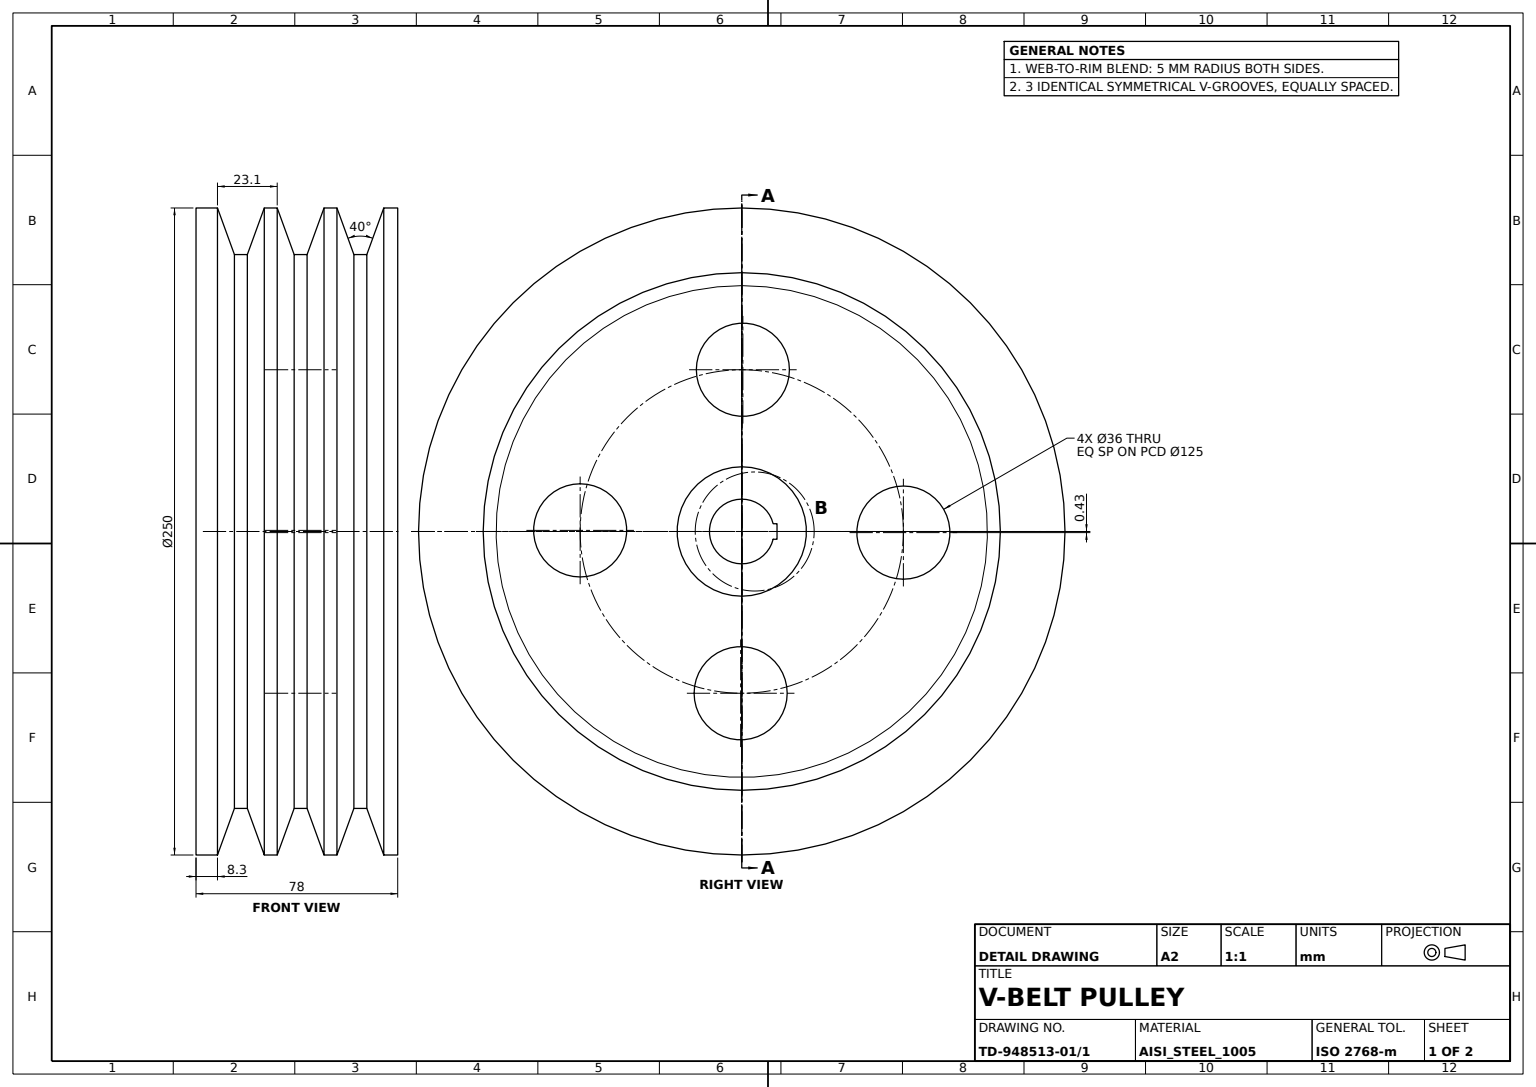
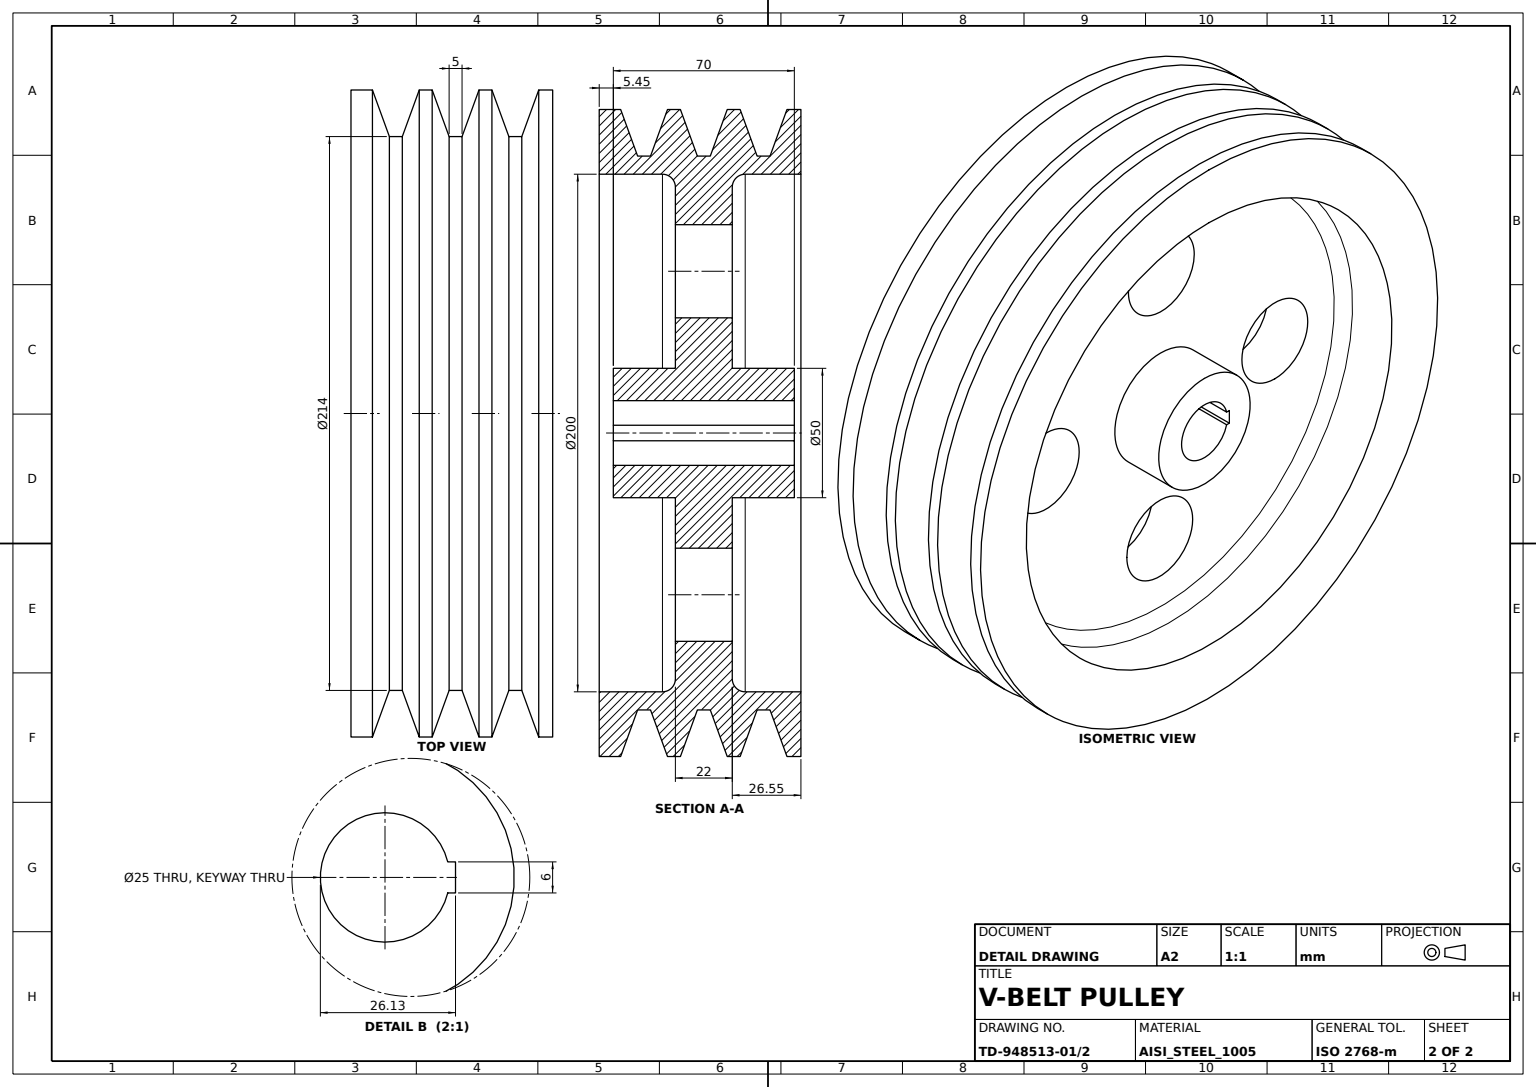
ISO-10303-21;
HEADER;
FILE_DESCRIPTION((''),'2;1');
FILE_NAME('','',(''),(''),'','','');
FILE_SCHEMA(('AUTOMOTIVE_DESIGN'));
ENDSEC;
DATA;
#1=APPLICATION_CONTEXT('');
#2=PRODUCT_CONTEXT('',#1,'mechanical');
#3=PRODUCT('','','',(#2));
#4=PRODUCT_DEFINITION_FORMATION('','',#3);
#5=PRODUCT_DEFINITION_CONTEXT('',#1,'design');
#6=PRODUCT_DEFINITION('','',#4,#5);
#7=PRODUCT_DEFINITION_SHAPE('','',#6);
#8=(LENGTH_UNIT()NAMED_UNIT(*)SI_UNIT(.MILLI.,.METRE.));
#9=(NAMED_UNIT(*)PLANE_ANGLE_UNIT()SI_UNIT($,.RADIAN.));
#10=(NAMED_UNIT(*)SI_UNIT($,.STERADIAN.)SOLID_ANGLE_UNIT());
#11=UNCERTAINTY_MEASURE_WITH_UNIT(LENGTH_MEASURE(0.005),#8,'distance_accuracy_value','');
#12=(GEOMETRIC_REPRESENTATION_CONTEXT(3)GLOBAL_UNCERTAINTY_ASSIGNED_CONTEXT((#11))GLOBAL_UNIT_ASSIGNED_CONTEXT((#8,#9,#10))REPRESENTATION_CONTEXT('',''));
#13=CARTESIAN_POINT('',(35.,12.134661,-3.));
#14=VERTEX_POINT('',#13);
#15=CARTESIAN_POINT('',(35.,13.634661,-3.));
#16=VERTEX_POINT('',#15);
#17=DIRECTION('',(0.,1.,0.));
#18=VECTOR('',#17,1000.);
#19=LINE('',#13,#18);
#20=EDGE_CURVE('',#14,#16,#19,.T.);
#21=ORIENTED_EDGE('',*,*,#20,.F.);
#22=CARTESIAN_POINT('',(35.,12.134661,3.));
#23=VERTEX_POINT('',#22);
#24=CARTESIAN_POINT('',(35.,0.,0.));
#25=DIRECTION('',(-1.,0.,0.));
#26=DIRECTION('',(0.,0.,1.));
#27=AXIS2_PLACEMENT_3D('',#24,#25,#26);
#28=CIRCLE('',#27,12.5);
#29=EDGE_CURVE('',#14,#23,#28,.T.);
#30=ORIENTED_EDGE('',*,*,#29,.T.);
#31=CARTESIAN_POINT('',(35.,13.634661,3.));
#32=VERTEX_POINT('',#31);
#33=DIRECTION('',(0.,-1.,0.));
#34=VECTOR('',#33,1000.);
#35=LINE('',#31,#34);
#36=EDGE_CURVE('',#32,#23,#35,.T.);
#37=ORIENTED_EDGE('',*,*,#36,.F.);
#38=VECTOR('',#26,1000.);
#39=LINE('',#15,#38);
#40=EDGE_CURVE('',#16,#32,#39,.T.);
#41=ORIENTED_EDGE('',*,*,#40,.F.);
#42=EDGE_LOOP('',(#21,#30,#37,#41));
#43=FACE_BOUND('',#42,.T.);
#44=CARTESIAN_POINT('',(35.,0.,25.));
#45=VERTEX_POINT('',#44);
#46=CIRCLE('',#27,25.);
#47=EDGE_CURVE('',#45,#45,#46,.T.);
#48=ORIENTED_EDGE('',*,*,#47,.F.);
#49=EDGE_LOOP('',(#48));
#50=FACE_BOUND('',#49,.T.);
#51=CARTESIAN_POINT('',(35.,12.5,0.));
#52=AXIS2_PLACEMENT_3D('',#51,#25,#26);
#53=PLANE('',#52);
#54=ADVANCED_FACE('',(#43,#50),#53,.F.);
#55=CARTESIAN_POINT('',(11.,0.,25.));
#56=VERTEX_POINT('',#55);
#57=CARTESIAN_POINT('',(11.,0.,0.));
#58=AXIS2_PLACEMENT_3D('',#57,#25,#26);
#59=CIRCLE('',#58,25.);
#60=EDGE_CURVE('',#56,#56,#59,.T.);
#61=ORIENTED_EDGE('',*,*,#60,.F.);
#62=EDGE_LOOP('',(#61));
#63=FACE_BOUND('',#62,.T.);
#64=ORIENTED_EDGE('',*,*,#47,.T.);
#65=EDGE_LOOP('',(#64));
#66=FACE_BOUND('',#65,.T.);
#67=CARTESIAN_POINT('',(0.,0.,0.));
#68=AXIS2_PLACEMENT_3D('',#67,#25,#26);
#69=CYLINDRICAL_SURFACE('',#68,25.);
#70=ADVANCED_FACE('',(#63,#66),#69,.T.);
#71=CARTESIAN_POINT('',(-35.,12.134661,-3.));
#72=VERTEX_POINT('',#71);
#73=VECTOR('',#25,1000.);
#74=LINE('',#13,#73);
#75=EDGE_CURVE('',#14,#72,#74,.T.);
#76=ORIENTED_EDGE('',*,*,#75,.F.);
#77=ORIENTED_EDGE('',*,*,#20,.T.);
#78=CARTESIAN_POINT('',(-35.,13.634661,-3.));
#79=VERTEX_POINT('',#78);
#80=LINE('',#15,#73);
#81=EDGE_CURVE('',#79,#16,#80,.F.);
#82=ORIENTED_EDGE('',*,*,#81,.F.);
#83=LINE('',#71,#18);
#84=EDGE_CURVE('',#72,#79,#83,.T.);
#85=ORIENTED_EDGE('',*,*,#84,.F.);
#86=EDGE_LOOP('',(#76,#77,#82,#85));
#87=FACE_BOUND('',#86,.T.);
#88=AXIS2_PLACEMENT_3D('',#13,#26,#33);
#89=PLANE('',#88);
#90=ADVANCED_FACE('',(#87),#89,.T.);
#91=CARTESIAN_POINT('',(-40.451548,0.,125.));
#92=VERTEX_POINT('',#91);
#93=CARTESIAN_POINT('',(-40.451548,0.,0.));
#94=AXIS2_PLACEMENT_3D('',#93,#25,#26);
#95=CIRCLE('',#94,125.);
#96=EDGE_CURVE('',#92,#92,#95,.T.);
#97=ORIENTED_EDGE('',*,*,#96,.T.);
#98=EDGE_LOOP('',(#97));
#99=FACE_BOUND('',#98,.T.);
#100=CARTESIAN_POINT('',(-40.451548,0.,100.));
#101=VERTEX_POINT('',#100);
#102=CIRCLE('',#94,100.);
#103=EDGE_CURVE('',#101,#101,#102,.T.);
#104=ORIENTED_EDGE('',*,*,#103,.F.);
#105=EDGE_LOOP('',(#104));
#106=FACE_BOUND('',#105,.T.);
#107=CARTESIAN_POINT('',(-40.451548,125.,0.));
#108=DIRECTION('',(1.,0.,0.));
#109=DIRECTION('',(0.,0.,-1.));
#110=AXIS2_PLACEMENT_3D('',#107,#108,#109);
#111=PLANE('',#110);
#112=ADVANCED_FACE('',(#99,#106),#111,.F.);
#113=CARTESIAN_POINT('',(16.,0.,100.));
#114=VERTEX_POINT('',#113);
#115=CARTESIAN_POINT('',(16.,0.,0.));
#116=AXIS2_PLACEMENT_3D('',#115,#25,#26);
#117=CIRCLE('',#116,100.);
#118=EDGE_CURVE('',#114,#114,#117,.T.);
#119=ORIENTED_EDGE('',*,*,#118,.T.);
#120=EDGE_LOOP('',(#119));
#121=FACE_BOUND('',#120,.T.);
#122=CARTESIAN_POINT('',(37.548452,0.,100.));
#123=VERTEX_POINT('',#122);
#124=CARTESIAN_POINT('',(37.548452,0.,0.));
#125=AXIS2_PLACEMENT_3D('',#124,#25,#26);
#126=CIRCLE('',#125,100.);
#127=EDGE_CURVE('',#123,#123,#126,.T.);
#128=ORIENTED_EDGE('',*,*,#127,.F.);
#129=EDGE_LOOP('',(#128));
#130=FACE_BOUND('',#129,.T.);
#131=CYLINDRICAL_SURFACE('',#68,100.);
#132=ADVANCED_FACE('',(#121,#130),#131,.F.);
#133=ORIENTED_EDGE('',*,*,#40,.T.);
#134=CARTESIAN_POINT('',(-35.,13.634661,3.));
#135=VERTEX_POINT('',#134);
#136=LINE('',#31,#73);
#137=EDGE_CURVE('',#135,#32,#136,.F.);
#138=ORIENTED_EDGE('',*,*,#137,.F.);
#139=LINE('',#78,#38);
#140=EDGE_CURVE('',#79,#135,#139,.T.);
#141=ORIENTED_EDGE('',*,*,#140,.F.);
#142=ORIENTED_EDGE('',*,*,#81,.T.);
#143=EDGE_LOOP('',(#133,#138,#141,#142));
#144=FACE_BOUND('',#143,.T.);
#145=AXIS2_PLACEMENT_3D('',#15,#33,#109);
#146=PLANE('',#145);
#147=ADVANCED_FACE('',(#144),#146,.T.);
#148=ORIENTED_EDGE('',*,*,#118,.F.);
#149=EDGE_LOOP('',(#148));
#150=FACE_BOUND('',#149,.T.);
#151=CARTESIAN_POINT('',(11.,0.,95.));
#152=VERTEX_POINT('',#151);
#153=CIRCLE('',#58,95.);
#154=EDGE_CURVE('',#152,#152,#153,.F.);
#155=ORIENTED_EDGE('',*,*,#154,.F.);
#156=EDGE_LOOP('',(#155));
#157=FACE_BOUND('',#156,.T.);
#158=TOROIDAL_SURFACE('',#116,95.,5.);
#159=ADVANCED_FACE('',(#150,#157),#158,.F.);
#160=CARTESIAN_POINT('',(-11.,-62.498511,-17.568647));
#161=VERTEX_POINT('',#160);
#162=CARTESIAN_POINT('',(-11.,-62.498511,0.431353));
#163=AXIS2_PLACEMENT_3D('',#162,#108,#109);
#164=CIRCLE('',#163,18.);
#165=EDGE_CURVE('',#161,#161,#164,.F.);
#166=ORIENTED_EDGE('',*,*,#165,.T.);
#167=EDGE_LOOP('',(#166));
#168=FACE_BOUND('',#167,.T.);
#169=CARTESIAN_POINT('',(11.,-62.498511,18.431353));
#170=VERTEX_POINT('',#169);
#171=CARTESIAN_POINT('',(11.,-62.498511,0.431353));
#172=AXIS2_PLACEMENT_3D('',#171,#25,#26);
#173=CIRCLE('',#172,18.);
#174=EDGE_CURVE('',#170,#170,#173,.T.);
#175=ORIENTED_EDGE('',*,*,#174,.F.);
#176=EDGE_LOOP('',(#175));
#177=FACE_BOUND('',#176,.T.);
#178=CARTESIAN_POINT('',(-9.,-62.498511,0.431353));
#179=AXIS2_PLACEMENT_3D('',#178,#25,#26);
#180=CYLINDRICAL_SURFACE('',#179,18.);
#181=ADVANCED_FACE('',(#168,#177),#180,.F.);
#182=CARTESIAN_POINT('',(25.602928,0.,107.));
#183=VERTEX_POINT('',#182);
#184=CARTESIAN_POINT('',(25.602928,0.,0.));
#185=AXIS2_PLACEMENT_3D('',#184,#25,#26);
#186=CIRCLE('',#185,107.);
#187=EDGE_CURVE('',#183,#183,#186,.T.);
#188=ORIENTED_EDGE('',*,*,#187,.T.);
#189=EDGE_LOOP('',(#188));
#190=FACE_BOUND('',#189,.T.);
#191=CARTESIAN_POINT('',(20.602928,0.,107.));
#192=VERTEX_POINT('',#191);
#193=CARTESIAN_POINT('',(20.602928,0.,0.));
#194=AXIS2_PLACEMENT_3D('',#193,#25,#26);
#195=CIRCLE('',#194,107.);
#196=EDGE_CURVE('',#192,#192,#195,.T.);
#197=ORIENTED_EDGE('',*,*,#196,.F.);
#198=EDGE_LOOP('',(#197));
#199=FACE_BOUND('',#198,.T.);
#200=CYLINDRICAL_SURFACE('',#68,107.);
#201=ADVANCED_FACE('',(#190,#199),#200,.T.);
#202=ORIENTED_EDGE('',*,*,#96,.F.);
#203=EDGE_LOOP('',(#202));
#204=FACE_BOUND('',#203,.T.);
#205=CARTESIAN_POINT('',(-32.154393,0.,125.));
#206=VERTEX_POINT('',#205);
#207=CARTESIAN_POINT('',(-32.154393,0.,0.));
#208=AXIS2_PLACEMENT_3D('',#207,#25,#26);
#209=CIRCLE('',#208,125.);
#210=EDGE_CURVE('',#206,#206,#209,.T.);
#211=ORIENTED_EDGE('',*,*,#210,.T.);
#212=EDGE_LOOP('',(#211));
#213=FACE_BOUND('',#212,.T.);
#214=CYLINDRICAL_SURFACE('',#68,125.);
#215=ADVANCED_FACE('',(#204,#213),#214,.T.);
#216=CARTESIAN_POINT('',(-16.,0.,-100.));
#217=VERTEX_POINT('',#216);
#218=CARTESIAN_POINT('',(-16.,0.,0.));
#219=AXIS2_PLACEMENT_3D('',#218,#108,#109);
#220=CIRCLE('',#219,100.);
#221=EDGE_CURVE('',#217,#217,#220,.T.);
#222=ORIENTED_EDGE('',*,*,#221,.F.);
#223=EDGE_LOOP('',(#222));
#224=FACE_BOUND('',#223,.T.);
#225=CARTESIAN_POINT('',(-11.,0.,-95.));
#226=VERTEX_POINT('',#225);
#227=CARTESIAN_POINT('',(-11.,0.,0.));
#228=AXIS2_PLACEMENT_3D('',#227,#108,#109);
#229=CIRCLE('',#228,95.);
#230=EDGE_CURVE('',#226,#226,#229,.F.);
#231=ORIENTED_EDGE('',*,*,#230,.F.);
#232=EDGE_LOOP('',(#231));
#233=FACE_BOUND('',#232,.T.);
#234=TOROIDAL_SURFACE('',#219,95.,5.);
#235=ADVANCED_FACE('',(#224,#233),#234,.F.);
#236=CARTESIAN_POINT('',(-9.051464,0.,125.));
#237=VERTEX_POINT('',#236);
#238=CARTESIAN_POINT('',(-9.051464,0.,0.));
#239=AXIS2_PLACEMENT_3D('',#238,#25,#26);
#240=CIRCLE('',#239,125.);
#241=EDGE_CURVE('',#237,#237,#240,.T.);
#242=ORIENTED_EDGE('',*,*,#241,.F.);
#243=EDGE_LOOP('',(#242));
#244=FACE_BOUND('',#243,.T.);
#245=CARTESIAN_POINT('',(-2.5,0.,107.));
#246=VERTEX_POINT('',#245);
#247=CARTESIAN_POINT('',(-2.5,0.,0.));
#248=AXIS2_PLACEMENT_3D('',#247,#25,#26);
#249=CIRCLE('',#248,107.);
#250=EDGE_CURVE('',#246,#246,#249,.T.);
#251=ORIENTED_EDGE('',*,*,#250,.T.);
#252=EDGE_LOOP('',(#251));
#253=FACE_BOUND('',#252,.T.);
#254=CONICAL_SURFACE('',#248,107.,1.221730476);
#255=ADVANCED_FACE('',(#244,#253),#254,.T.);
#256=CARTESIAN_POINT('',(37.548452,0.,125.));
#257=VERTEX_POINT('',#256);
#258=CIRCLE('',#125,125.);
#259=EDGE_CURVE('',#257,#257,#258,.T.);
#260=ORIENTED_EDGE('',*,*,#259,.T.);
#261=EDGE_LOOP('',(#260));
#262=FACE_BOUND('',#261,.T.);
#263=CARTESIAN_POINT('',(32.154393,0.,125.));
#264=VERTEX_POINT('',#263);
#265=CARTESIAN_POINT('',(32.154393,0.,0.));
#266=AXIS2_PLACEMENT_3D('',#265,#25,#26);
#267=CIRCLE('',#266,125.);
#268=EDGE_CURVE('',#264,#264,#267,.T.);
#269=ORIENTED_EDGE('',*,*,#268,.F.);
#270=EDGE_LOOP('',(#269));
#271=FACE_BOUND('',#270,.T.);
#272=ADVANCED_FACE('',(#262,#271),#214,.T.);
#273=ORIENTED_EDGE('',*,*,#29,.F.);
#274=ORIENTED_EDGE('',*,*,#75,.T.);
#275=CARTESIAN_POINT('',(-35.,12.134661,3.));
#276=VERTEX_POINT('',#275);
#277=CARTESIAN_POINT('',(-35.,0.,0.));
#278=AXIS2_PLACEMENT_3D('',#277,#25,#26);
#279=CIRCLE('',#278,12.5);
#280=EDGE_CURVE('',#72,#276,#279,.T.);
#281=ORIENTED_EDGE('',*,*,#280,.T.);
#282=LINE('',#22,#73);
#283=EDGE_CURVE('',#23,#276,#282,.T.);
#284=ORIENTED_EDGE('',*,*,#283,.F.);
#285=EDGE_LOOP('',(#273,#274,#281,#284));
#286=FACE_BOUND('',#285,.T.);
#287=CYLINDRICAL_SURFACE('',#68,12.5);
#288=ADVANCED_FACE('',(#286),#287,.F.);
#289=CARTESIAN_POINT('',(14.051464,0.,125.));
#290=VERTEX_POINT('',#289);
#291=CARTESIAN_POINT('',(14.051464,0.,0.));
#292=AXIS2_PLACEMENT_3D('',#291,#25,#26);
#293=CIRCLE('',#292,125.);
#294=EDGE_CURVE('',#290,#290,#293,.T.);
#295=ORIENTED_EDGE('',*,*,#294,.F.);
#296=EDGE_LOOP('',(#295));
#297=FACE_BOUND('',#296,.T.);
#298=ORIENTED_EDGE('',*,*,#196,.T.);
#299=EDGE_LOOP('',(#298));
#300=FACE_BOUND('',#299,.T.);
#301=CONICAL_SURFACE('',#194,107.,1.221730476);
#302=ADVANCED_FACE('',(#297,#300),#301,.T.);
#303=CARTESIAN_POINT('',(9.051464,0.,125.));
#304=VERTEX_POINT('',#303);
#305=CARTESIAN_POINT('',(9.051464,0.,0.));
#306=AXIS2_PLACEMENT_3D('',#305,#25,#26);
#307=CIRCLE('',#306,125.);
#308=EDGE_CURVE('',#304,#304,#307,.T.);
#309=ORIENTED_EDGE('',*,*,#308,.F.);
#310=EDGE_LOOP('',(#309));
#311=FACE_BOUND('',#310,.T.);
#312=ORIENTED_EDGE('',*,*,#294,.T.);
#313=EDGE_LOOP('',(#312));
#314=FACE_BOUND('',#313,.T.);
#315=ADVANCED_FACE('',(#311,#314),#214,.T.);
#316=ORIENTED_EDGE('',*,*,#127,.T.);
#317=EDGE_LOOP('',(#316));
#318=FACE_BOUND('',#317,.T.);
#319=ORIENTED_EDGE('',*,*,#259,.F.);
#320=EDGE_LOOP('',(#319));
#321=FACE_BOUND('',#320,.T.);
#322=CARTESIAN_POINT('',(37.548452,100.,0.));
#323=AXIS2_PLACEMENT_3D('',#322,#25,#26);
#324=PLANE('',#323);
#325=ADVANCED_FACE('',(#318,#321),#324,.F.);
#326=ORIENTED_EDGE('',*,*,#241,.T.);
#327=EDGE_LOOP('',(#326));
#328=FACE_BOUND('',#327,.T.);
#329=CARTESIAN_POINT('',(-14.051464,0.,125.));
#330=VERTEX_POINT('',#329);
#331=CARTESIAN_POINT('',(-14.051464,0.,0.));
#332=AXIS2_PLACEMENT_3D('',#331,#25,#26);
#333=CIRCLE('',#332,125.);
#334=EDGE_CURVE('',#330,#330,#333,.T.);
#335=ORIENTED_EDGE('',*,*,#334,.F.);
#336=EDGE_LOOP('',(#335));
#337=FACE_BOUND('',#336,.T.);
#338=ADVANCED_FACE('',(#328,#337),#214,.T.);
#339=CARTESIAN_POINT('',(11.,-18.431353,-62.498511));
#340=VERTEX_POINT('',#339);
#341=CARTESIAN_POINT('',(11.,-0.431353,-62.498511));
#342=AXIS2_PLACEMENT_3D('',#341,#25,#33);
#343=CIRCLE('',#342,18.);
#344=EDGE_CURVE('',#340,#340,#343,.T.);
#345=ORIENTED_EDGE('',*,*,#344,.F.);
#346=EDGE_LOOP('',(#345));
#347=FACE_BOUND('',#346,.T.);
#348=CARTESIAN_POINT('',(-11.,-0.431353,-80.498511));
#349=VERTEX_POINT('',#348);
#350=CARTESIAN_POINT('',(-11.,-0.431353,-62.498511));
#351=AXIS2_PLACEMENT_3D('',#350,#108,#109);
#352=CIRCLE('',#351,18.);
#353=EDGE_CURVE('',#349,#349,#352,.F.);
#354=ORIENTED_EDGE('',*,*,#353,.T.);
#355=EDGE_LOOP('',(#354));
#356=FACE_BOUND('',#355,.T.);
#357=CARTESIAN_POINT('',(-9.,-0.431353,-62.498511));
#358=AXIS2_PLACEMENT_3D('',#357,#25,#26);
#359=CYLINDRICAL_SURFACE('',#358,18.);
#360=ADVANCED_FACE('',(#347,#356),#359,.F.);
#361=CARTESIAN_POINT('',(-11.,0.431353,44.498511));
#362=VERTEX_POINT('',#361);
#363=CARTESIAN_POINT('',(-11.,0.431353,62.498511));
#364=AXIS2_PLACEMENT_3D('',#363,#108,#109);
#365=CIRCLE('',#364,18.);
#366=EDGE_CURVE('',#362,#362,#365,.F.);
#367=ORIENTED_EDGE('',*,*,#366,.F.);
#368=EDGE_LOOP('',(#367));
#369=FACE_BOUND('',#368,.T.);
#370=ORIENTED_EDGE('',*,*,#165,.F.);
#371=EDGE_LOOP('',(#370));
#372=FACE_BOUND('',#371,.T.);
#373=ORIENTED_EDGE('',*,*,#353,.F.);
#374=EDGE_LOOP('',(#373));
#375=FACE_BOUND('',#374,.T.);
#376=CARTESIAN_POINT('',(-11.,62.498511,-18.431353));
#377=VERTEX_POINT('',#376);
#378=CARTESIAN_POINT('',(-11.,62.498511,-0.431353));
#379=AXIS2_PLACEMENT_3D('',#378,#108,#109);
#380=CIRCLE('',#379,18.);
#381=EDGE_CURVE('',#377,#377,#380,.F.);
#382=ORIENTED_EDGE('',*,*,#381,.F.);
#383=EDGE_LOOP('',(#382));
#384=FACE_BOUND('',#383,.T.);
#385=ORIENTED_EDGE('',*,*,#230,.T.);
#386=EDGE_LOOP('',(#385));
#387=FACE_BOUND('',#386,.T.);
#388=CARTESIAN_POINT('',(-11.,0.,25.));
#389=VERTEX_POINT('',#388);
#390=AXIS2_PLACEMENT_3D('',#227,#25,#26);
#391=CIRCLE('',#390,25.);
#392=EDGE_CURVE('',#389,#389,#391,.T.);
#393=ORIENTED_EDGE('',*,*,#392,.F.);
#394=EDGE_LOOP('',(#393));
#395=FACE_BOUND('',#394,.T.);
#396=CARTESIAN_POINT('',(-11.,100.,0.));
#397=AXIS2_PLACEMENT_3D('',#396,#108,#109);
#398=PLANE('',#397);
#399=ADVANCED_FACE('',(#369,#372,#375,#384,#387,#395),#398,.F.);
#400=ORIENTED_EDGE('',*,*,#308,.T.);
#401=EDGE_LOOP('',(#400));
#402=FACE_BOUND('',#401,.T.);
#403=CARTESIAN_POINT('',(2.5,0.,107.));
#404=VERTEX_POINT('',#403);
#405=CARTESIAN_POINT('',(2.5,0.,0.));
#406=AXIS2_PLACEMENT_3D('',#405,#25,#26);
#407=CIRCLE('',#406,107.);
#408=EDGE_CURVE('',#404,#404,#407,.T.);
#409=ORIENTED_EDGE('',*,*,#408,.F.);
#410=EDGE_LOOP('',(#409));
#411=FACE_BOUND('',#410,.T.);
#412=AXIS2_PLACEMENT_3D('',#305,#108,#109);
#413=CONICAL_SURFACE('',#412,125.,1.221730476);
#414=ADVANCED_FACE('',(#402,#411),#413,.T.);
#415=CARTESIAN_POINT('',(-25.602928,0.,107.));
#416=VERTEX_POINT('',#415);
#417=CARTESIAN_POINT('',(-25.602928,0.,0.));
#418=AXIS2_PLACEMENT_3D('',#417,#25,#26);
#419=CIRCLE('',#418,107.);
#420=EDGE_CURVE('',#416,#416,#419,.T.);
#421=ORIENTED_EDGE('',*,*,#420,.T.);
#422=EDGE_LOOP('',(#421));
#423=FACE_BOUND('',#422,.T.);
#424=ORIENTED_EDGE('',*,*,#210,.F.);
#425=EDGE_LOOP('',(#424));
#426=FACE_BOUND('',#425,.T.);
#427=CONICAL_SURFACE('',#418,107.,1.221730476);
#428=ADVANCED_FACE('',(#423,#426),#427,.T.);
#429=ORIENTED_EDGE('',*,*,#103,.T.);
#430=EDGE_LOOP('',(#429));
#431=FACE_BOUND('',#430,.T.);
#432=ORIENTED_EDGE('',*,*,#221,.T.);
#433=EDGE_LOOP('',(#432));
#434=FACE_BOUND('',#433,.T.);
#435=ADVANCED_FACE('',(#431,#434),#131,.F.);
#436=ORIENTED_EDGE('',*,*,#366,.T.);
#437=EDGE_LOOP('',(#436));
#438=FACE_BOUND('',#437,.T.);
#439=CARTESIAN_POINT('',(11.,18.431353,62.498511));
#440=VERTEX_POINT('',#439);
#441=CARTESIAN_POINT('',(11.,0.431353,62.498511));
#442=AXIS2_PLACEMENT_3D('',#441,#25,#17);
#443=CIRCLE('',#442,18.);
#444=EDGE_CURVE('',#440,#440,#443,.T.);
#445=ORIENTED_EDGE('',*,*,#444,.F.);
#446=EDGE_LOOP('',(#445));
#447=FACE_BOUND('',#446,.T.);
#448=CARTESIAN_POINT('',(-9.,0.431353,62.498511));
#449=AXIS2_PLACEMENT_3D('',#448,#25,#26);
#450=CYLINDRICAL_SURFACE('',#449,18.);
#451=ADVANCED_FACE('',(#438,#447),#450,.F.);
#452=CARTESIAN_POINT('',(-20.602928,0.,107.));
#453=VERTEX_POINT('',#452);
#454=CARTESIAN_POINT('',(-20.602928,0.,0.));
#455=AXIS2_PLACEMENT_3D('',#454,#25,#26);
#456=CIRCLE('',#455,107.);
#457=EDGE_CURVE('',#453,#453,#456,.T.);
#458=ORIENTED_EDGE('',*,*,#457,.F.);
#459=EDGE_LOOP('',(#458));
#460=FACE_BOUND('',#459,.T.);
#461=ORIENTED_EDGE('',*,*,#334,.T.);
#462=EDGE_LOOP('',(#461));
#463=FACE_BOUND('',#462,.T.);
#464=AXIS2_PLACEMENT_3D('',#331,#108,#109);
#465=CONICAL_SURFACE('',#464,125.,1.221730476);
#466=ADVANCED_FACE('',(#460,#463),#465,.T.);
#467=ORIENTED_EDGE('',*,*,#174,.T.);
#468=EDGE_LOOP('',(#467));
#469=FACE_BOUND('',#468,.T.);
#470=ORIENTED_EDGE('',*,*,#60,.T.);
#471=EDGE_LOOP('',(#470));
#472=FACE_BOUND('',#471,.T.);
#473=ORIENTED_EDGE('',*,*,#344,.T.);
#474=EDGE_LOOP('',(#473));
#475=FACE_BOUND('',#474,.T.);
#476=ORIENTED_EDGE('',*,*,#444,.T.);
#477=EDGE_LOOP('',(#476));
#478=FACE_BOUND('',#477,.T.);
#479=ORIENTED_EDGE('',*,*,#154,.T.);
#480=EDGE_LOOP('',(#479));
#481=FACE_BOUND('',#480,.T.);
#482=CARTESIAN_POINT('',(11.,62.498511,-18.431353));
#483=VERTEX_POINT('',#482);
#484=CARTESIAN_POINT('',(11.,62.498511,-0.431353));
#485=AXIS2_PLACEMENT_3D('',#484,#25,#109);
#486=CIRCLE('',#485,18.);
#487=EDGE_CURVE('',#483,#483,#486,.T.);
#488=ORIENTED_EDGE('',*,*,#487,.T.);
#489=EDGE_LOOP('',(#488));
#490=FACE_BOUND('',#489,.T.);
#491=CARTESIAN_POINT('',(11.,25.,0.));
#492=AXIS2_PLACEMENT_3D('',#491,#25,#26);
#493=PLANE('',#492);
#494=ADVANCED_FACE('',(#469,#472,#475,#478,#481,#490),#493,.F.);
#495=CARTESIAN_POINT('',(-35.,0.,25.));
#496=VERTEX_POINT('',#495);
#497=CIRCLE('',#278,25.);
#498=EDGE_CURVE('',#496,#496,#497,.T.);
#499=ORIENTED_EDGE('',*,*,#498,.T.);
#500=EDGE_LOOP('',(#499));
#501=FACE_BOUND('',#500,.T.);
#502=ORIENTED_EDGE('',*,*,#140,.T.);
#503=LINE('',#134,#34);
#504=EDGE_CURVE('',#135,#276,#503,.T.);
#505=ORIENTED_EDGE('',*,*,#504,.T.);
#506=ORIENTED_EDGE('',*,*,#280,.F.);
#507=ORIENTED_EDGE('',*,*,#84,.T.);
#508=EDGE_LOOP('',(#502,#505,#506,#507));
#509=FACE_BOUND('',#508,.T.);
#510=CARTESIAN_POINT('',(-35.,25.,0.));
#511=AXIS2_PLACEMENT_3D('',#510,#108,#109);
#512=PLANE('',#511);
#513=ADVANCED_FACE('',(#501,#509),#512,.F.);
#514=ORIENTED_EDGE('',*,*,#408,.T.);
#515=EDGE_LOOP('',(#514));
#516=FACE_BOUND('',#515,.T.);
#517=ORIENTED_EDGE('',*,*,#250,.F.);
#518=EDGE_LOOP('',(#517));
#519=FACE_BOUND('',#518,.T.);
#520=ADVANCED_FACE('',(#516,#519),#200,.T.);
#521=ORIENTED_EDGE('',*,*,#392,.T.);
#522=EDGE_LOOP('',(#521));
#523=FACE_BOUND('',#522,.T.);
#524=ORIENTED_EDGE('',*,*,#498,.F.);
#525=EDGE_LOOP('',(#524));
#526=FACE_BOUND('',#525,.T.);
#527=ADVANCED_FACE('',(#523,#526),#69,.T.);
#528=ORIENTED_EDGE('',*,*,#457,.T.);
#529=EDGE_LOOP('',(#528));
#530=FACE_BOUND('',#529,.T.);
#531=ORIENTED_EDGE('',*,*,#420,.F.);
#532=EDGE_LOOP('',(#531));
#533=FACE_BOUND('',#532,.T.);
#534=ADVANCED_FACE('',(#530,#533),#200,.T.);
#535=ORIENTED_EDGE('',*,*,#487,.F.);
#536=EDGE_LOOP('',(#535));
#537=FACE_BOUND('',#536,.T.);
#538=ORIENTED_EDGE('',*,*,#381,.T.);
#539=EDGE_LOOP('',(#538));
#540=FACE_BOUND('',#539,.T.);
#541=CARTESIAN_POINT('',(-9.,62.498511,-0.431353));
#542=AXIS2_PLACEMENT_3D('',#541,#25,#26);
#543=CYLINDRICAL_SURFACE('',#542,18.);
#544=ADVANCED_FACE('',(#537,#540),#543,.F.);
#545=ORIENTED_EDGE('',*,*,#36,.T.);
#546=ORIENTED_EDGE('',*,*,#283,.T.);
#547=ORIENTED_EDGE('',*,*,#504,.F.);
#548=ORIENTED_EDGE('',*,*,#137,.T.);
#549=EDGE_LOOP('',(#545,#546,#547,#548));
#550=FACE_BOUND('',#549,.T.);
#551=AXIS2_PLACEMENT_3D('',#31,#109,#17);
#552=PLANE('',#551);
#553=ADVANCED_FACE('',(#550),#552,.T.);
#554=ORIENTED_EDGE('',*,*,#268,.T.);
#555=EDGE_LOOP('',(#554));
#556=FACE_BOUND('',#555,.T.);
#557=ORIENTED_EDGE('',*,*,#187,.F.);
#558=EDGE_LOOP('',(#557));
#559=FACE_BOUND('',#558,.T.);
#560=AXIS2_PLACEMENT_3D('',#265,#108,#109);
#561=CONICAL_SURFACE('',#560,125.,1.221730476);
#562=ADVANCED_FACE('',(#556,#559),#561,.T.);
#563=CLOSED_SHELL('',(#54,#70,#90,#112,#132,#147,#159,#181,#201,#215,#235,#255,#272,#288,#302,#315,#325,#338,#360,#399,#414,#428,#435,#451,#466,#494,#513,#520,#527,#534,#544,#553,#562));
#564=MANIFOLD_SOLID_BREP('',#563);
#565=ADVANCED_BREP_SHAPE_REPRESENTATION('',(#564),#12);
#566=SHAPE_DEFINITION_REPRESENTATION(#7,#565);
ENDSEC;
END-ISO-10303-21;
